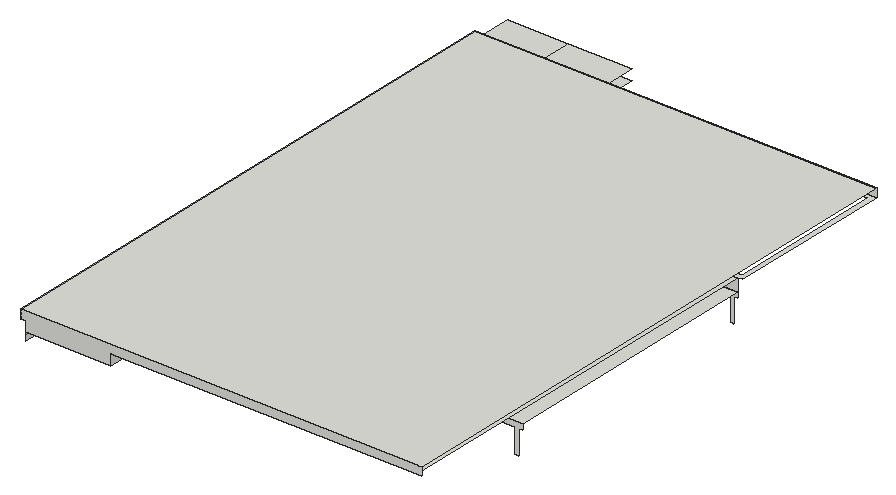
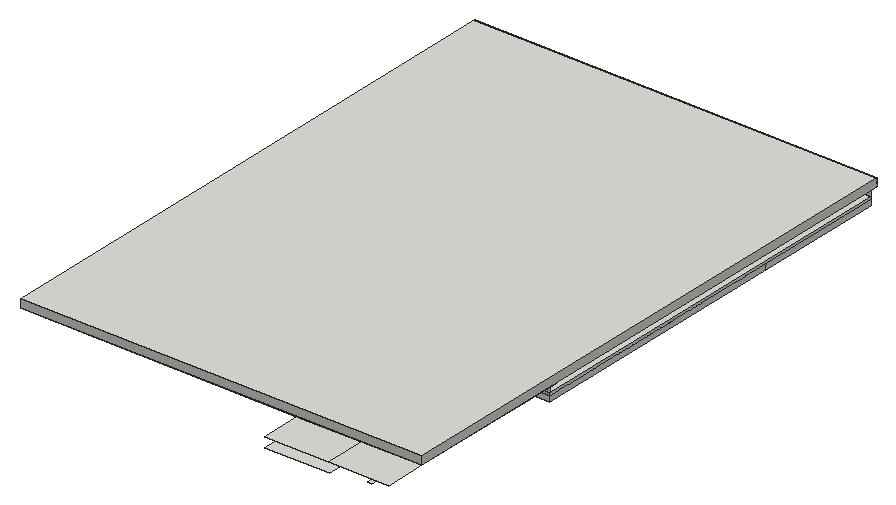
# SketchUp Ruby script. Lengths in inches.
U = 1.inch
M = Sketchup.active_model
def pt(a) = Geom::Point3d.new(a.map { |v| v * U })
def face(e, loops, mat)
  f = e.add_face(loops[0].map { |a| pt(a) })
  loops[1..].each { |l| e.add_face(l.map { |a| pt(a) }).erase! }
  f.material = f.back_material = mat if mat
  f
end
# faces: each face lists its corners as indices into pts; further lists are holes
def faces(e, pts, list, mat = nil) = list.each { |f| face(e, (f[0].is_a?(Array) ? f : [f]).map { |l| l.map { |i| pts[i] } }, mat) }
# xy, xz, yz: faces in a plane at the given z, y or x. An outline is a flat list of corners, or four numbers for a rectangle; further outlines are holes
def ring(l) = l.size == 4 ? [[l[0], l[1]], [l[2], l[1]], [l[2], l[3]], [l[0], l[3]]] : l.each_slice(2).to_a
def flat(e, list, mat, &to3) = list.each { |f| face(e, (f[0].is_a?(Array) ? f : [f]).map { |l| ring(l).map { |u, v| to3.(u, v) } }, mat) }
def xy(e, z, list, mat = nil) = flat(e, list, mat) { |x, y| [x, y, z] }
def xz(e, y, list, mat = nil) = flat(e, list, mat) { |x, z| [x, y, z] }
def yz(e, x, list, mat = nil) = flat(e, list, mat) { |y, z| [x, y, z] }
def lines(e, pts, list) = list.each { |a, b| e.add_line(pt(pts[a]), pt(pts[b])) }
# prism: a flat outline (further loops are holes) pulled along v
def prism(e, loops, v, mat = nil)
  f = face(e, loops, mat); d = Geom::Vector3d.new(v.map { |x| x * U })
  f.pushpull(f.normal.samedirection?(d) ? d.length : -d.length)
end
def box(e, o, s, mat = nil) = prism(e, [[o, [o[0] + s[0], o[1], o[2]], [o[0] + s[0], o[1] + s[1], o[2]], [o[0], o[1] + s[1], o[2]]]], [0, 0, s[2]], mat)
def at(x, y, z, deg = 0) = Geom::Transformation.translation(pt([x, y, z])) * Geom::Transformation.rotation(ORIGIN, Z_AXIS, deg.degrees)
def axes(o, x, y, z) = Geom::Transformation.new([*x, 0, *y, 0, *z, 0, *pt(o).to_a, 1])
def part(name) = M.definitions.add(name)
# library, detail: a bought-in or finely detailed component or shape, given as its bounding box
def library(name, o, s) = part(name).tap { |d| box(d.entities, o, s) }
def detail(e, o, s) = box(e.add_group.entities, o, s)
def put(e, d, t, mat = nil) = e.add_instance(d, t).tap { |i| i.material = mat if mat }
def group(e, t, mat = nil) = e.add_group.tap { |g| g.transformation = t; g.material = mat if mat }.entities
root = M.entities
M.materials.add("[0129_WhiteSmoke]").color = [255, 255, 255]
c1 = library("10 (1)",[26.65,-5.45,122.92],[1.37,1.38,0.36])
c2 = library("031_FANZART_Zen",[-27.59,-27.12,5.07],[46.53,51.77,17.09])
xy(root,93.25,[[41.22,302.6,44.125,342.1]])
xy(root,93.9375,[[41.22,394.68,44.125,412.06]])
xy(root,109.39,[[101.71,131.9375,102.71,132.9375],[115.71,144.9375,143.02,145.9375],[143.02,144.9375,173.19,145.9375],[101.71,258.91,102.71,259.91],[102.71,258.91,114.71,259.91],
  [114.71,258.91,115.71,259.91],[105.89,294.47,109.17,294.91],[129.06,294.47,132.13,294.91],[178,294.47,181.65,294.91],[182.38,294.47,186.03,294.91],
  [186.75,294.47,190.4,294.91],[191.13,294.47,194.78,294.91],[195.5,294.47,199.15,294.91],[199.88,294.47,203.53,294.91],[204.25,294.47,207.9,294.91],
  [208.63,294.47,212.28,294.91],[213,294.47,216.65,294.91],[217.38,294.47,221.03,294.91],[221.75,294.47,225.4,294.91]])
xy(root,109.39,[[3.79,96.9375,66.71,294.91],[[66.71,96.9375,66.71,294.91,105.89,294.91,105.89,294.47,109.17,294.47,109.17,294.91,129.06,294.91,129.06,294.47,132.13,294.47,132.13,294.91,178,294.91,178,294.47,181.65,294.47,181.65,294.91,182.38,294.91,182.38,294.47,186.03,294.47,186.03,294.91,186.75,294.91,186.75,294.47,190.4,294.47,190.4,294.91,191.13,294.91,191.13,294.47,194.78,294.47,194.78,294.91,195.5,294.91,195.5,294.47,199.15,294.47,199.15,294.91,199.88,294.91,199.88,294.47,203.53,294.47,203.53,294.91,204.25,294.91,204.25,294.47,207.9,294.47,207.9,294.91,208.63,294.91,208.63,294.47,212.28,294.47,212.28,294.91,213,294.91,213,294.47,216.65,294.47,216.65,294.91,217.38,294.91,217.38,294.47,221.03,294.47,221.03,294.91,221.75,294.91,221.75,294.47,225.4,294.47,225.4,294.91,255.93,294.91,255.93,294.47,260.26,294.47,260.26,294.91,260.79,294.91,260.79,294.47,264.44,294.47,264.44,294.91,264.79,294.91,264.79,294.47,266.48,294.47,266.48,294.91,266.83,294.91,266.83,294.47,268.52,294.47,268.52,294.91,268.86,294.91,268.86,294.47,270.55,294.47,270.55,294.91,270.9,294.91,270.9,294.47,272.59,294.47,272.59,294.91,272.94,294.91,272.94,294.47,274.63,294.47,274.63,294.91,274.98,294.91,274.98,294.47,276.67,294.47,276.67,294.91,277.02,294.91,277.02,294.47,278.7,294.47,278.7,294.91,286.12,294.91,286.12,96.9375],[101.71,131.9375,256.63,259.91],[83.71,191.92,84.74,192.06,85.71,192.46,86.54,193.09,87.17,193.92,87.57,194.89,87.71,195.92,87.57,196.96,87.17,197.92,86.54,198.75,85.71,199.39,84.74,199.79,83.71,199.92,82.67,199.79,81.71,199.39,80.88,198.75,80.24,197.92,79.84,196.96,79.71,195.92,79.84,194.89,80.24,193.92,80.88,193.09,81.71,192.46,82.67,192.06],[274.63,191.92,275.67,192.06,276.63,192.46,277.46,193.09,278.09,193.92,278.49,194.89,278.63,195.92,278.49,196.96,278.09,197.92,277.46,198.75,276.63,199.39,275.67,199.79,274.63,199.92,273.6,199.79,272.63,199.39,271.8,198.75,271.17,197.92,270.77,196.96,270.63,195.92,270.77,194.89,271.17,193.92,271.8,193.09,272.63,192.46,273.6,192.06],[119.71,109.9375,120.74,110.07,121.71,110.47,122.54,111.11,123.17,111.9375,123.57,112.9,123.71,113.9375,123.57,114.97,123.17,115.9375,122.54,116.77,121.71,117.4,120.74,117.8,119.71,117.9375,118.67,117.8,117.71,117.4,116.88,116.77,116.24,115.9375,115.84,114.97,115.71,113.9375,115.84,112.9,116.24,111.9375,116.88,111.11,117.71,110.47,118.67,110.07],[238.63,109.9375,239.67,110.07,240.63,110.47,241.46,111.11,242.09,111.9375,242.49,112.9,242.63,113.9375,242.49,114.97,242.09,115.9375,241.46,116.77,240.63,117.4,239.67,117.8,238.63,117.9375,237.6,117.8,236.63,117.4,235.8,116.77,235.17,115.9375,234.77,114.97,234.63,113.9375,234.77,112.9,235.17,111.9375,235.8,111.11,236.63,110.47,237.6,110.07],[238.63,273.91,239.67,274.04,240.63,274.44,241.46,275.08,242.09,275.91,242.49,276.87,242.63,277.91,242.49,278.94,242.09,279.91,241.46,280.73,240.63,281.37,239.67,281.77,238.63,281.91,237.6,281.77,236.63,281.37,235.8,280.73,235.17,279.91,234.77,278.94,234.63,277.91,234.77,276.87,235.17,275.91,235.8,275.08,236.63,274.44,237.6,274.04],[119.71,273.91,120.74,274.04,121.71,274.44,122.54,275.08,123.17,275.91,123.57,276.87,123.71,277.91,123.57,278.94,123.17,279.91,122.54,280.73,121.71,281.37,120.74,281.77,119.71,281.91,118.67,281.77,117.71,281.37,116.88,280.73,116.24,279.91,115.84,278.94,115.71,277.91,115.84,276.87,116.24,275.91,116.88,275.08,117.71,274.44,118.67,274.04]],[[102.71,132.9375,255.63,258.91],[114.71,145.9375,115.71,145.9375,115.71,183.89,114.71,183.89,114.71,246.91,176.41,246.91,176.41,245.91,224.48,245.91,224.48,246.91,114.71,246.91],[143.02,144.9375,243.63,144.9375,243.63,246.91,242.63,246.91,242.63,211.08,243.63,211.08,243.63,144.9375,173.19,144.9375,173.19,145.9375,143.02,145.9375]]],"[0129_WhiteSmoke]")
xy(root,109.96,[[114.71,144.9375,115.71,145.9375],[114.71,145.9375,115.71,183.89],[176.41,245.91,224.48,246.91],[115.71,258.91,255.63,259.91]])
xy(root,110.08,[[102.71,131.9375,255.63,132.9375],[101.71,132.9375,102.71,258.91]])
xy(root,110.77,[[119.71,109.9375,118.67,110.07,117.71,110.47,116.88,111.11,116.24,111.9375,115.84,112.9,115.71,113.9375,115.84,114.97,116.24,115.9375,116.88,116.77,117.71,117.4,118.67,117.8,119.71,117.9375,120.74,117.8,121.71,117.4,122.54,116.77,123.17,115.9375,123.57,114.97,123.71,113.9375,123.57,112.9,123.17,111.9375,122.54,111.11,121.71,110.47,120.74,110.07],[83.71,191.92,82.67,192.06,81.71,192.46,80.88,193.09,80.24,193.92,79.84,194.89,79.71,195.92,79.84,196.96,80.24,197.92,80.88,198.75,81.71,199.39,82.67,199.79,83.71,199.92,84.74,199.79,85.71,199.39,86.54,198.75,87.17,197.92,87.57,196.96,87.71,195.92,87.57,194.89,87.17,193.92,86.54,193.09,85.71,192.46,84.74,192.06],[119.71,273.91,118.67,274.04,117.71,274.44,116.88,275.08,116.24,275.91,115.84,276.87,115.71,277.91,115.84,278.94,116.24,279.91,116.88,280.73,117.71,281.37,118.67,281.77,119.71,281.91,120.74,281.77,121.71,281.37,122.54,280.73,123.17,279.91,123.57,278.94,123.71,277.91,123.57,276.87,123.17,275.91,122.54,275.08,121.71,274.44,120.74,274.04]])
xy(root,113.39,[[3.79,96.9375,66.71,294.91],[66.71,96.9375,291.63,294.91]])
xy(root,115.375,[[3.79,0,3.79,294.91,44.125,294.91,44.125,412.06,91.5625,412.06,91.5625,294.91,66.71,294.91,66.71,0],[44.125,412.06,91.5625,447.375]])
xy(root,123.125,[[66.71,0,291.63,294.91],[[0,294.91,44.125,417.6875],[2.9,297.81,41.22,414.79]],[91.5625,294.91,291.63,294.91,291.63,298.46,95.12,298.46,95.12,414.13,291.63,414.13,291.63,294.91,295.1875,294.91,295.1875,417.6875,91.5625,417.6875],[44.125,412.06,91.5625,417.6875],[0,417.6875,44.125,447.875],
  [44.125,417.6875,91.5625,447.875]])
xy(root,129.125,[[0,0,295.1875,417.6875]])
xz(root,0,[[3.79,115.375,66.71,115.375,66.71,123.125,295.1875,123.125,295.1875,129.125,0,129.125,0,123.125,3.79,123.125]])
xz(root,96.9375,[[286.12,91.83,289,91.83,289,109.39,291.63,109.39,291.63,113.39,66.71,113.39,66.71,109.39,286.12,109.39],[3.79,109.39,66.71,113.39]])
xz(root,131.9375,[[102.71,109.39,255.63,110.08]])
xz(root,132.9375,[[101.71,109.39,102.71,110.08],[102.71,109.39,255.63,110.08]])
xz(root,144.9375,[[114.71,109.39,115.71,109.96]])
xz(root,145.9375,[[114.71,109.39,115.71,109.96]])
xz(root,183.89,[[114.71,109.39,115.71,109.96]])
xz(root,245.91,[[176.41,109.39,224.48,109.96]])
xz(root,246.91,[[176.41,109.39,224.48,109.96]])
xz(root,258.91,[[101.71,109.39,102.71,110.08],[115.71,109.39,255.63,109.96]])
xz(root,259.91,[[115.71,109.39,255.63,109.96]])
xz(root,294.91,[[286.12,91.83,286.12,109.39,91.5625,109.39,91.5625,113.39,291.63,113.39,291.63,109.39,289,109.39,289,91.83],[3.79,109.39,44.125,113.39],[44.125,109.39,66.71,113.39],[66.71,109.39,91.5625,113.39],[3.79,113.39,44.125,115.375],
  [91.5625,113.39,291.63,123.125],[3.79,115.375,44.125,123.125],[66.71,115.375,91.5625,123.125]])
xz(root,412.06,[[44.125,115.375,91.5625,123.125]])
xz(root,417.6875,[[0,123.125,295.1875,129.125]])
yz(root,0,[[0,123.125,417.6875,129.125]])
yz(root,3.79,[[0,109.39,96.9375,113.39],[96.9375,109.39,294.91,113.39],[0,113.39,294.91,115.375]])
yz(root,44.125,[[294.91,115.375,412.06,123.125]])
yz(root,66.71,[[96.9375,109.39,294.91,113.39],[0,115.375,294.91,123.125]])
yz(root,91.5625,[[294.91,115.375,412.06,123.125],[412.06,115.375,417.6875,123.125]])
yz(root,101.71,[[132.9375,109.39,258.91,110.08]])
yz(root,102.71,[[131.9375,109.39,132.9375,110.08],[132.9375,109.39,258.91,110.08]])
yz(root,114.71,[[144.9375,109.39,145.9375,109.96],[145.9375,109.39,183.89,109.96]])
yz(root,115.71,[[144.9375,109.39,145.9375,109.96],[145.9375,109.39,183.89,109.96],[258.91,109.39,259.91,109.96]])
yz(root,176.41,[[245.91,109.39,246.91,109.96]])
yz(root,224.48,[[245.91,109.39,246.91,109.96]])
yz(root,225.4,[[294.47,89.72,294.91,109.39]])
p = [[226.39,293.53,88.86],[226.39,294.66,88.86],[227.05,294.66,89.43],[227.05,293.53,89.43],[227.05,294.91,89.43],[227.17,294.91,89.53],
  [227.17,294.66,89.53],[230.15,294.66,92.0625],[230.15,293.53,92.0625],[225.94,294.91,90.31],[225.4,294.91,89.72],[225.4,294.47,89.72],
  [225.4,293.53,89.72],[225.94,293.53,90.31],[226.51,294.91,90.875],[226.51,293.53,90.875],[227.1,294.91,91.41],[227.1,293.53,91.41],
  [227.71,294.91,91.93],[227.71,293.53,91.93],[228.35,294.91,92.42],[228.35,293.53,92.42],[230.15,294.91,92.0625],[230.375,294.91,92.16],
  [230.375,294.66,92.16],[233.34,294.66,93.47],[233.34,293.53,93.47],[229,294.91,92.875],[229,293.53,92.875],[229.68,294.91,93.31],
  [229.68,293.53,93.31],[230.37,294.91,93.71],[230.37,293.53,93.71],[231.08,294.91,94.08],[231.08,293.53,94.08],[231.8,294.91,94.42],
  [231.8,293.53,94.42],[232.54,294.91,94.73],[232.54,293.53,94.73],[233.29,294.91,95],[233.29,293.53,95],[119.71,109.9375,109.39],
  [118.67,110.07,109.39],[118.67,110.07,110.77],[119.71,109.9375,110.77],[120.74,110.07,109.39],[120.74,110.07,110.77],[117.71,110.47,109.39],
  [117.71,110.47,110.77],[121.71,110.47,109.39],[121.71,110.47,110.77],[116.88,111.11,109.39],[116.88,111.11,110.77],[122.54,111.11,109.39],
  [122.54,111.11,110.77],[116.24,111.9375,109.39],[116.24,111.9375,110.77],[123.17,111.9375,109.39],[123.17,111.9375,110.77],[115.84,112.9,109.39],
  [115.84,112.9,110.77],[123.57,112.9,109.39],[123.57,112.9,110.77],[115.71,113.9375,109.39],[115.71,113.9375,110.77],[123.71,113.9375,109.39],
  [123.71,113.9375,110.77],[115.84,114.97,109.39],[115.84,114.97,110.77],[123.57,114.97,109.39],[123.57,114.97,110.77],[116.24,115.9375,109.39],
  [116.24,115.9375,110.77],[123.17,115.9375,109.39],[123.17,115.9375,110.77],[116.88,116.77,109.39],[116.88,116.77,110.77],[122.54,116.77,109.39],
  [122.54,116.77,110.77],[117.71,117.4,109.39],[117.71,117.4,110.77],[121.71,117.4,109.39],[121.71,117.4,110.77],[118.67,117.8,109.39],
  [118.67,117.8,110.77],[120.74,117.8,109.39],[120.74,117.8,110.77],[119.71,117.9375,109.39],[119.71,117.9375,110.77],[83.71,191.92,109.39],
  [82.67,192.06,109.39],[82.67,192.06,110.77],[83.71,191.92,110.77],[84.74,192.06,109.39],[84.74,192.06,110.77],[81.71,192.46,109.39],
  [81.71,192.46,110.77],[85.71,192.46,109.39],[85.71,192.46,110.77],[80.88,193.09,109.39],[80.88,193.09,110.77],[86.54,193.09,109.39],
  [86.54,193.09,110.77],[80.24,193.92,109.39],[80.24,193.92,110.77],[87.17,193.92,109.39],[87.17,193.92,110.77],[79.84,194.89,109.39],
  [79.84,194.89,110.77],[87.57,194.89,109.39],[87.57,194.89,110.77],[79.71,195.92,109.39],[79.71,195.92,110.77],[87.71,195.92,109.39],
  [87.71,195.92,110.77],[79.84,196.96,109.39],[79.84,196.96,110.77],[87.57,196.96,109.39],[87.57,196.96,110.77],[80.24,197.92,109.39],
  [80.24,197.92,110.77],[87.17,197.92,109.39],[87.17,197.92,110.77],[80.88,198.75,109.39],[80.88,198.75,110.77],[86.54,198.75,109.39],
  [86.54,198.75,110.77],[81.71,199.39,109.39],[81.71,199.39,110.77],[85.71,199.39,109.39],[85.71,199.39,110.77],[82.67,199.79,109.39],
  [82.67,199.79,110.77],[84.74,199.79,109.39],[84.74,199.79,110.77],[83.71,199.92,109.39],[83.71,199.92,110.77],[119.71,273.91,109.39],
  [118.67,274.04,109.39],[118.67,274.04,110.77],[119.71,273.91,110.77],[120.74,274.04,109.39],[120.74,274.04,110.77],[117.71,274.44,109.39],
  [117.71,274.44,110.77],[121.71,274.44,109.39],[121.71,274.44,110.77],[116.88,275.08,109.39],[116.88,275.08,110.77],[122.54,275.08,109.39],
  [122.54,275.08,110.77],[116.24,275.91,109.39],[116.24,275.91,110.77],[123.17,275.91,109.39],[123.17,275.91,110.77],[115.84,276.87,109.39],
  [115.84,276.87,110.77],[123.57,276.87,109.39],[123.57,276.87,110.77],[115.71,277.91,109.39],[115.71,277.91,110.77],[123.71,277.91,109.39],
  [123.71,277.91,110.77],[115.84,278.94,109.39],[115.84,278.94,110.77],[123.57,278.94,109.39],[123.57,278.94,110.77],[116.24,279.91,109.39],
  [116.24,279.91,110.77],[123.17,279.91,109.39],[123.17,279.91,110.77],[116.88,280.73,109.39],[116.88,280.73,110.77],[122.54,280.73,109.39],
  [122.54,280.73,110.77],[117.71,281.37,109.39],[117.71,281.37,110.77],[121.71,281.37,109.39],[121.71,281.37,110.77],[118.67,281.77,109.39],
  [118.67,281.77,110.77],[120.74,281.77,109.39],[120.74,281.77,110.77],[119.71,281.91,109.39],[119.71,281.91,110.77]]
faces(root,p,[[0,1,2,3],[4,5,6,7,8,3,2],[9,10,11,12,13],[14,9,13,15],[16,14,15,17],[18,16,17,19],[20,18,19,21],[22,23,24,25,26,8,7],
  [27,20,21,28],[29,27,28,30],[31,29,30,32],[33,31,32,34],[35,33,34,36],[37,35,36,38],[39,37,38,40],[41,42,43,44],
  [45,41,44,46],[42,47,48,43],[49,45,46,50],[47,51,52,48],[53,49,50,54],[51,55,56,52],[57,53,54,58],[55,59,60,56],
  [61,57,58,62],[59,63,64,60],[65,61,62,66],[63,67,68,64],[69,65,66,70],[67,71,72,68],[73,69,70,74],[71,75,76,72],
  [77,73,74,78],[75,79,80,76],[81,77,78,82],[79,83,84,80],[85,81,82,86],[83,87,88,84],[87,85,86,88],[89,90,91,92],
  [93,89,92,94],[90,95,96,91],[97,93,94,98],[95,99,100,96],[101,97,98,102],[99,103,104,100],[105,101,102,106],[103,107,108,104],
  [109,105,106,110],[107,111,112,108],[113,109,110,114],[111,115,116,112],[117,113,114,118],[115,119,120,116],[121,117,118,122],[119,123,124,120],
  [125,121,122,126],[123,127,128,124],[129,125,126,130],[127,131,132,128],[133,129,130,134],[131,135,136,132],[135,133,134,136],[137,138,139,140],
  [141,137,140,142],[138,143,144,139],[145,141,142,146],[143,147,148,144],[149,145,146,150],[147,151,152,148],[153,149,150,154],[151,155,156,152],
  [157,153,154,158],[155,159,160,156],[161,157,158,162],[159,163,164,160],[165,161,162,166],[163,167,168,164],[169,165,166,170],[167,171,172,168],
  [173,169,170,174],[171,175,176,172],[177,173,174,178],[175,179,180,176],[181,177,178,182],[179,183,184,180],[183,181,182,184]])
put(root,c1,axes([-93.62,225.8125,-1587.85],[6.49609,0,0],[0,6.19526,0],[0,0,13.8072]))
put(root,c1,axes([-58.23,144.11,-1588.37],[6.49609,0,0],[0,6.19526,0],[0,0,13.8072]))
put(root,c1,axes([-57.95,307.48,-1589.04],[6.49609,0,0],[0,6.19526,0],[0,0,13.8072]))
put(root,c2,axes([183.99,188.84,94.29],[1,0,0],[0,1,0],[0,0,0.7502]))
